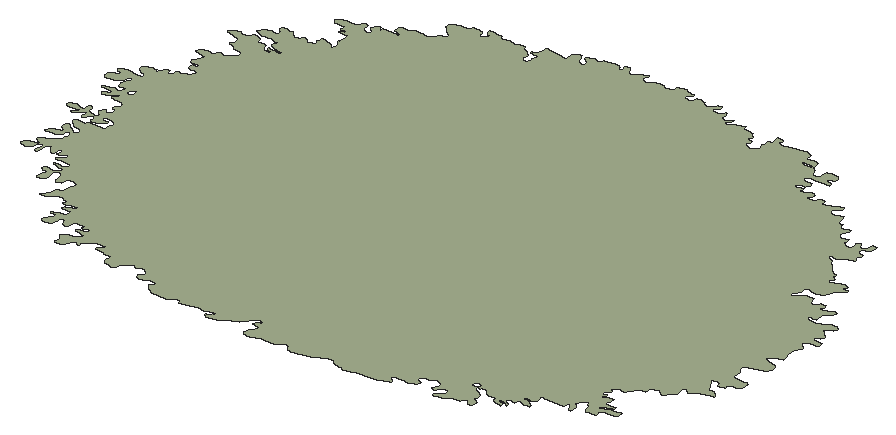
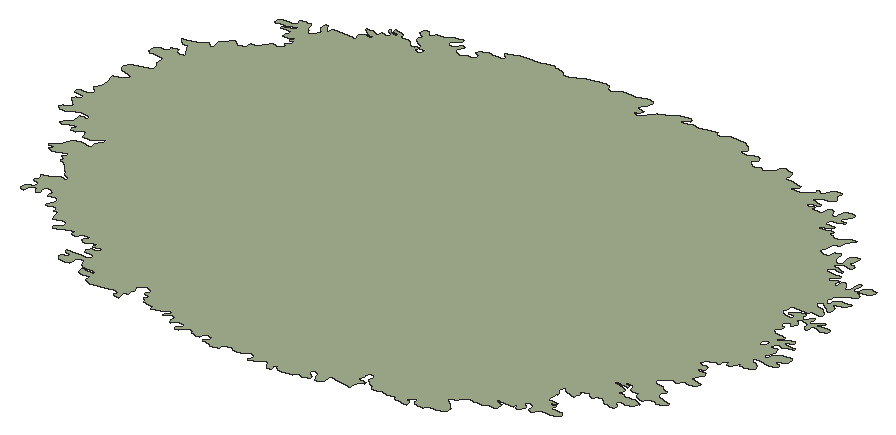
# SketchUp Ruby script. Lengths in inches.
U = 1.inch
M = Sketchup.active_model
def pt(a) = Geom::Point3d.new(a.map { |v| v * U })
def face(e, loops, mat)
  f = e.add_face(loops[0].map { |a| pt(a) })
  loops[1..].each { |l| e.add_face(l.map { |a| pt(a) }).erase! }
  f.material = f.back_material = mat if mat
  f
end
# faces: each face lists its corners as indices into pts; further lists are holes
def faces(e, pts, list, mat = nil) = list.each { |f| face(e, (f[0].is_a?(Array) ? f : [f]).map { |l| l.map { |i| pts[i] } }, mat) }
# xy, xz, yz: faces in a plane at the given z, y or x. An outline is a flat list of corners, or four numbers for a rectangle; further outlines are holes
def ring(l) = l.size == 4 ? [[l[0], l[1]], [l[2], l[1]], [l[2], l[3]], [l[0], l[3]]] : l.each_slice(2).to_a
def flat(e, list, mat, &to3) = list.each { |f| face(e, (f[0].is_a?(Array) ? f : [f]).map { |l| ring(l).map { |u, v| to3.(u, v) } }, mat) }
def xy(e, z, list, mat = nil) = flat(e, list, mat) { |x, y| [x, y, z] }
def xz(e, y, list, mat = nil) = flat(e, list, mat) { |x, z| [x, y, z] }
def yz(e, x, list, mat = nil) = flat(e, list, mat) { |y, z| [x, y, z] }
def lines(e, pts, list) = list.each { |a, b| e.add_line(pt(pts[a]), pt(pts[b])) }
# prism: a flat outline (further loops are holes) pulled along v
def prism(e, loops, v, mat = nil)
  f = face(e, loops, mat); d = Geom::Vector3d.new(v.map { |x| x * U })
  f.pushpull(f.normal.samedirection?(d) ? d.length : -d.length)
end
def box(e, o, s, mat = nil) = prism(e, [[o, [o[0] + s[0], o[1], o[2]], [o[0] + s[0], o[1] + s[1], o[2]], [o[0], o[1] + s[1], o[2]]]], [0, 0, s[2]], mat)
def at(x, y, z, deg = 0) = Geom::Transformation.translation(pt([x, y, z])) * Geom::Transformation.rotation(ORIGIN, Z_AXIS, deg.degrees)
def axes(o, x, y, z) = Geom::Transformation.new([*x, 0, *y, 0, *z, 0, *pt(o).to_a, 1])
def part(name) = M.definitions.add(name)
# library, detail: a bought-in or finely detailed component or shape, given as its bounding box
def library(name, o, s) = part(name).tap { |d| box(d.entities, o, s) }
def detail(e, o, s) = box(e.add_group.entities, o, s)
def put(e, d, t, mat = nil) = e.add_instance(d, t).tap { |i| i.material = mat if mat }
def group(e, t, mat = nil) = e.add_group.tap { |g| g.transformation = t; g.material = mat if mat }.entities
root = M.entities
M.materials.add("Boxwoodplan").color = [166, 177, 144]
xy(root,9.058,[[[245.938,66.701,245.827,66.705,245.732,66.73,245.676,66.786,245.675,66.889,245.701,66.953,245.764,67.016,245.813,67.08,245.872,67.177,245.685,67.207,245.595,67.216,245.615,67.304,245.701,67.362,245.732,67.372,245.727,67.417,245.638,67.449,245.522,67.408,245.425,67.278,245.283,67.123,245.122,67.036,245.016,67.013,244.956,66.988,244.94,66.945,244.795,66.853,244.602,66.822,244.513,66.831,244.432,66.878,244.432,66.899,244.478,66.93,244.568,67.008,244.637,67.055,244.547,67.069,244.435,67.052,244.315,67.007,244.121,67.025,244.024,67.018,243.898,66.974,243.697,66.928,243.608,66.92,243.57,67.014,243.5625,67.036,243.495,67.044,243.406,67.026,243.238,66.908,243.038,66.899,242.808,66.924,242.641,67.018,242.499,67.181,242.682,67.274,242.583,67.327,242.447,67.344,242.32,67.321,242.248,67.268,242.168,67.244,242.052,67.309,242.01,67.377,242.097,67.418,242.124,67.479,242.129,67.529,242.088,67.581,242.015,67.657,241.93,67.689,241.843,67.635,241.776,67.61,241.72,67.652,241.704,67.675,241.68,67.693,241.65,67.683,241.571,67.629,241.499,67.581,241.423,67.495,241.412,67.362,241.34,67.32,241.29,67.294,241.23,67.297,241.131,67.317,241.045,67.365,241.001,67.433,240.992,67.522,241.001,67.589,241.014,67.611,240.995,67.651,240.782,67.671,240.85,67.707,240.823,67.708,240.731,67.702,240.561,67.718,240.484,67.744,240.467,67.778,240.481,67.796,240.607,67.885,240.604,67.942,240.52,67.965,240.36,67.961,240.23,67.891,240.132,67.805,240.058,67.77,240.01,67.744,240.009,67.725,240.046,67.673,240.03,67.617,239.959,67.653,239.896,67.692,239.834,67.644,239.812,67.589,239.781,67.475,239.733,67.427,239.66,67.393,239.569,67.387,239.499,67.413,239.481,67.446,239.488,67.464,239.509,67.504,239.531,67.563,239.5,67.62,239.399,67.721,239.513,67.801,239.574,67.841,239.653,67.856,239.721,67.887,239.776,67.941,239.86,68.048,239.789,68.074,239.709,68.082,239.577,68.102,239.538,68.137,239.546,68.156,239.62,68.191,239.782,68.229,239.825,68.28,239.82,68.319,239.794,68.335,239.644,68.282,239.598,68.304,239.599,68.323,239.621,68.386,239.46,68.397,239.38,68.405,239.326,68.397,239.318,68.378,239.302,68.281,239.287,68.214,239.246,68.163,239.199,68.15,239.179,68.165,239.12,68.211,239.076,68.329,239.036,68.355,239.009,68.356,238.956,68.348,238.949,68.329,238.947,68.213,238.892,68.095,238.832,68.021,238.752,67.991,238.673,67.994,238.626,68.019,238.593,68.078,238.594,68.135,238.647,68.248,238.761,68.356,238.782,68.374,238.768,68.394,238.742,68.4,238.661,68.418,238.581,68.431,238.554,68.447,238.56,68.466,238.581,68.485,238.729,68.553,238.891,68.577,238.933,68.679,238.907,68.74,238.86,68.762,238.832,68.758,238.669,68.74,238.629,68.771,238.635,68.791,238.663,68.85,238.82,68.905,238.992,68.975,239.041,69.014,239.027,69.035,238.931,69.008,238.759,68.989,238.615,68.943,238.526,68.957,238.499,68.963,238.506,68.983,238.526,68.998,238.581,69.042,238.554,69.079,238.526,69.075,238.444,69.083,238.389,69.131,238.375,69.173,238.347,69.169,238.265,69.146,238.108,69.06,237.958,68.984,237.884,68.952,237.829,68.964,237.842,68.984,237.862,69.024,237.888,69.041,237.913,69.121,237.962,69.222,237.994,69.33,238.045,69.384,238.119,69.423,238.163,69.544,238.185,69.684,238.204,69.798,238.2,69.857,238.155,69.893,238.075,69.906,237.988,69.906,237.915,69.881,237.905,69.817,237.905,69.755,237.872,69.696,237.784,69.659,237.728,69.668,237.689,69.727,237.679,69.788,237.653,69.909,237.647,69.971,237.607,70.025,237.579,70.047,237.542,70.0625,237.483,70.051,237.448,70.031,237.447,70,237.439,69.938,237.441,69.801,237.466,69.739,237.458,69.675,237.408,69.61,237.359,69.582,237.321,69.57,237.284,69.575,237.242,69.583,237.224,69.61,237.22,69.738,237.241,69.795,237.286,69.848,237.302,69.878,237.293,69.906,237.236,69.911,237.155,69.918,237.117,69.933,237.094,69.962,237.091,70.024,237.107,70.055,237.141,70.071,237.314,70.043,237.392,70.068,237.442,70.098,237.502,70.145,237.516,70.208,237.493,70.234,237.449,70.235,237.371,70.242,237.279,70.253,237.178,70.289,237.16,70.318,237.165,70.332,237.185,70.335,237.244,70.347,237.42,70.333,237.509,70.358,237.522,70.415,237.496,70.478,237.424,70.518,237.345,70.524,237.231,70.518,237.132,70.492,237.048,70.51,237.044,70.54,237.065,70.568,237.111,70.625,237.178,70.682,237.231,70.762,237.222,70.796,237.178,70.8125,237.113,70.811,236.995,70.711,236.955,70.713,236.921,70.733,236.942,70.792,236.959,70.859,236.915,70.921,236.875,70.938,236.855,70.939,236.85,70.924,236.854,70.878,236.851,70.735,236.81,70.674,236.77,70.679,236.736,70.703,236.638,70.834,236.613,70.899,236.589,70.926,236.573,70.915,236.518,70.865,236.483,70.806,236.502,70.675,236.507,70.608,236.487,70.543,236.438,70.534,236.403,70.55,236.393,70.594,236.413,70.726,236.423,70.804,236.423,70.842,236.408,70.854,236.393,70.843,236.313,70.809,236.274,70.754,236.264,70.691,236.225,70.649,236.088,70.558,236.049,70.549,236.004,70.558,235.925,70.598,235.904,70.628,235.908,70.661,235.941,70.722,236.039,70.808,236.128,70.835,236.218,70.835,236.313,70.839,236.253,70.89,236.101,70.975,236.085,71.037,236.138,71.075,236.229,71.144,236.348,71.206,236.467,71.281,236.502,71.294,236.528,71.318,236.555,71.361,236.558,71.453,236.59,71.574,236.591,71.636,236.57,71.657,236.549,71.666,236.486,71.681,236.452,71.676,236.449,71.66,236.46,71.567,236.419,71.506,236.371,71.47,236.293,71.442,236.222,71.43,236.062,71.405,236.027,71.41,236.013,71.424,236.014,71.432,236.022,71.472,236.039,71.518,236.081,71.566,236.151,71.613,236.209,71.635,236.268,71.637,236.306,71.639,236.326,71.647,236.349,71.668,236.345,71.692,236.29,71.723,236.222,71.779,236.19,71.836,236.186,71.903,236.199,71.953,236.252,71.998,236.278,72.003,236.289,71.996,236.308,71.983,236.351,71.922,236.4,71.876,236.529,71.798,236.602,71.764,236.638,71.748,236.658,71.756,236.682,71.777,236.688,71.794,236.7,71.835,236.684,71.892,236.642,71.938,236.609,71.961,236.576,71.973,236.516,71.973,236.442,71.976,236.398,72.018,236.312,72.09,236.253,72.141,236.214,72.188,236.215,72.217,236.239,72.243,236.296,72.27,236.331,72.275,236.372,72.271,236.432,72.251,236.493,72.249,236.529,72.256,236.564,72.297,236.612,72.328,236.672,72.336,236.743,72.335,236.896,72.343,237.037,72.363,237.069,72.38,237.07,72.397,237.064,72.44,237.053,72.484,237.064,72.528,237.094,72.632,237.08,72.655,237.058,72.668,237.001,72.698,236.947,72.735,236.875,72.763,236.802,72.766,236.751,72.756,236.73,72.742,236.705,72.69,236.71,72.669,236.722,72.665,236.745,72.66,236.896,72.648,236.922,72.642,236.928,72.634,236.918,72.618,236.878,72.578,236.833,72.535,236.768,72.499,236.707,72.455,236.634,72.42,236.597,72.424,236.577,72.435,236.552,72.471,236.545,72.567,236.528,72.592,236.546,72.606,236.553,72.649,236.547,72.659,236.535,72.66,236.521,72.658,236.495,72.655,236.462,72.648,236.445,72.636,236.363,72.541,236.332,72.486,236.3,72.463,236.278,72.466,236.252,72.487,236.243,72.504,236.237,72.544,236.265,72.629,236.271,72.674,236.262,72.701,236.241,72.708,236.203,72.699,236.183,72.686,236.137,72.636,236.016,72.529,235.979,72.504,235.954,72.499,235.916,72.506,235.904,72.523,235.996,72.629,236.058,72.674,236.072,72.7,236.072,72.717,236.063,72.724,236.051,72.72,236.037,72.714,236.005,72.703,235.922,72.679,235.754,72.661,235.681,72.668,235.634,72.693,235.612,72.72,235.611,72.737,235.628,72.789,235.675,72.835,235.736,72.852,235.806,72.856,235.881,72.838,236.008,72.795,236.094,72.768,236.106,72.772,236.106,72.781,236.105,72.791,236.096,72.811,236.072,72.858,236.07,72.914,236.078,72.979,236.089,73.009,236.107,73.021,236.155,72.984,236.195,72.935,236.222,72.889,236.231,72.827,236.243,72.775,236.258,72.747,236.282,72.746,236.416,72.729,236.489,72.715,236.524,72.712,236.542,72.726,236.558,72.774,236.502,72.816,236.444,72.88,236.426,72.907,236.426,72.924,236.46,73.032,236.49,73.055,236.518,73.06,236.532,73.049,236.541,73.031,236.57,72.986,236.582,72.961,236.594,72.963,236.615,72.975,236.695,73.053,236.711,73.099,236.713,73.151,236.699,73.183,236.678,73.195,236.614,73.218,236.575,73.237,236.566,73.258,236.582,73.308,236.638,73.345,236.673,73.367,236.686,73.387,236.693,73.441,236.692,73.488,236.596,73.563,236.453,73.585,236.39,73.602,236.356,73.584,236.327,73.586,236.258,73.603,236.239,73.63,236.249,73.654,236.375,73.756,236.368,73.789,236.346,73.804,236.302,73.796,236.273,73.787,236.147,73.726,236.107,73.679,236.057,73.635,235.988,73.62,235.96,73.621,235.913,73.673,235.941,73.698,235.959,73.737,235.991,73.76,236.084,73.791,236.129,73.821,236.119,73.852,236.106,73.855,236.096,73.848,236.07,73.841,236.03,73.844,235.895,73.856,235.749,73.884,235.725,73.899,235.73,73.918,235.755,73.947,235.968,74.007,236.032,74.006,236.092,73.99,236.153,73.962,236.179,73.964,236.186,73.974,236.235,74.052,236.258,74.067,236.265,74.086,236.264,74.129,236.264,74.154,236.254,74.164,236.24,74.162,236.183,74.163,236.125,74.156,236.078,74.139,236.054,74.147,236.033,74.168,236.009,74.201,235.989,74.289,235.999,74.378,236.029,74.42,236.035,74.452,236.048,74.494,236.086,74.515,236.081,74.562,236.059,74.598,235.97,74.575,235.953,74.541,235.954,74.521,235.957,74.458,235.876,74.411,235.735,74.317,235.58,74.271,235.496,74.297,235.454,74.35,235.444,74.476,235.573,74.561,235.655,74.575,235.699,74.599,235.723,74.633,235.721,74.653,235.636,74.684,235.5625,74.71,235.5,74.766,235.536,74.82,235.612,74.849,235.708,74.883,235.773,74.882,235.951,74.839,236.043,74.817,236.128,74.821,236.179,74.84,236.185,74.861,236.17,74.927,236.109,74.979,236.064,74.986,235.952,75.057,235.905,75.099,235.89,75.135,235.884,75.189,235.884,75.216,235.897,75.231,235.939,75.266,235.99,75.281,236.104,75.312,236.134,75.322,236.175,75.321,236.225,75.317,236.237,75.305,236.252,75.275,236.267,75.261,236.276,75.261,236.305,75.264,236.321,75.276,236.341,75.326,236.369,75.359,236.386,75.382,236.388,75.407,236.405,75.432,236.424,75.444,236.472,75.456,236.511,75.448,236.533,75.404,236.537,75.353,236.553,75.326,236.575,75.326,236.616,75.367,236.641,75.41,236.656,75.514,236.671,75.539,236.704,75.546,236.735,75.546,236.755,75.534,236.776,75.512,236.808,75.511,236.86,75.533,236.905,75.579,236.918,75.603,236.908,75.617,236.968,75.615,236.996,75.618,237.012,75.637,237.017,75.686,237.051,75.726,237.086,75.772,237.032,75.815,236.964,75.844,236.927,75.842,236.895,75.832,236.852,75.821,236.811,75.827,236.789,75.843,236.767,75.866,236.744,75.969,236.757,75.994,236.763,76.011,236.773,76.014,236.877,76.035,236.923,76.043,236.942,76.054,236.932,76.058,236.846,76.086,236.78,76.098,236.752,76.091,236.716,76.091,236.68,76.092,236.645,76.104,236.606,76.154,236.588,76.183,236.588,76.213,236.604,76.235,236.632,76.25,236.664,76.269,236.672,76.296,236.701,76.354,236.729,76.408,236.735,76.461,236.727,76.488,236.687,76.499,236.609,76.525,236.436,76.572,236.401,76.59,236.384,76.614,236.419,76.668,236.464,76.703,236.509,76.73,236.564,76.75,236.617,76.759,236.669,76.756,236.724,76.732,236.78,76.734,236.806,76.738,236.819,76.759,236.837,76.8,236.874,76.836,236.894,76.854,236.921,76.856,236.99,76.839,237.052,76.828,237.078,76.825,237.102,76.84,237.188,76.907,237.276,76.972,237.329,77.069,237.326,77.114,237.284,77.15,237.167,77.188,237.042,77.218,236.955,77.291,236.898,77.326,236.829,77.347,236.801,77.359,236.788,77.38,236.81,77.426,236.858,77.468,236.856,77.553,236.806,77.631,236.676,77.6875,236.436,77.767,236.387,77.784,236.367,77.818,236.438,77.882,236.559,77.933,236.665,77.938,236.722,77.925,236.766,77.899,236.814,77.889,236.867,77.897,236.928,77.909,236.958,77.94,236.972,78.019,236.99,78.054,237.043,78.053,237.1,78.043,237.148,78.023,237.215,77.964,237.24,77.929,237.254,77.889,237.255,77.821,237.261,77.816,237.269,77.82,237.296,77.834,237.348,77.84,237.436,77.842,237.516,77.806,237.551,77.742,237.575,77.664,237.645,77.619,237.686,77.606,237.703,77.606,237.73,77.615,237.826,77.621,237.842,77.626,237.822,77.643,237.759,77.666,237.708,77.671,237.669,77.689,237.65,77.724,237.647,77.736,237.651,77.755,237.666,77.763,237.7,77.763,237.742,77.756,237.849,77.728,237.963,77.723,238.015,77.731,238.034,77.733,238.06,77.745,238.016,77.775,237.974,77.785,237.888,77.799,237.83,77.813,237.79,77.816,237.767,77.82,237.742,77.834,237.691,77.86,237.643,77.887,237.621,77.919,237.632,77.975,237.66,78.014,237.701,78.043,237.661,78.074,237.606,78.089,237.564,78.092,237.508,78.1,237.477,78.126,237.46,78.163,237.445,78.172,237.417,78.171,237.301,78.143,237.249,78.129,237.199,78.13,237.152,78.133,237.102,78.15,237.054,78.167,237.014,78.174,236.971,78.198,236.928,78.221,236.954,78.234,236.955,78.241,236.967,78.281,236.982,78.317,237.008,78.354,237.039,78.386,237.083,78.411,237.136,78.433,237.182,78.445,237.288,78.439,237.365,78.433,237.398,78.429,237.408,78.429,237.408,78.442,237.4,78.483,237.379,78.528,237.343,78.567,237.301,78.598,237.268,78.644,237.27,78.668,237.28,78.688,237.328,78.718,237.38,78.741,237.406,78.741,237.432,78.735,237.487,78.719,237.554,78.714,237.602,78.699,237.625,78.686,237.644,78.667,237.687,78.626,237.726,78.591,237.771,78.56,237.828,78.547,237.881,78.552,237.927,78.581,237.958,78.617,238.007,78.655,238.033,78.655,238.056,78.64,238.096,78.598,238.143,78.565,238.271,78.59,238.346,78.609,238.387,78.637,238.393,78.657,238.371,78.673,238.32,78.695,238.311,78.718,238.319,78.741,238.334,78.785,238.341,78.845,238.345,78.87,238.368,78.886,238.396,78.888,238.426,78.879,238.468,78.86,238.602,78.82,238.662,78.798,238.702,78.765,238.728,78.725,238.743,78.702,238.75,78.694,238.76,78.698,238.767,78.703,238.8,78.748,238.806,78.783,238.796,78.886,238.775,78.934,238.75,78.968,238.715,79.008,238.705,79.037,238.717,79.049,238.728,79.046,238.749,79.048,238.748,79.056,238.754,79.079,238.746,79.121,238.732,79.277,238.734,79.354,238.618,79.373,238.521,79.376,238.459,79.384,238.441,79.391,238.427,79.401,238.44,79.411,238.553,79.453,238.587,79.482,238.587,79.495,238.564,79.519,238.528,79.523,238.475,79.512,238.427,79.49,238.409,79.49,238.394,79.517,238.421,79.6,238.423,79.64,238.423,79.654,238.399,79.675,238.31,79.657,238.197,79.66,238.087,79.676,238.026,79.757,238.024,79.784,238.062,79.821,238.159,79.875,238.207,79.901,238.262,79.907,238.386,79.904,238.478,79.908,238.537,79.917,238.577,79.955,238.617,79.99,238.625,80.033,238.652,80.072,238.707,80.085,238.745,80.08,238.788,80.046,238.799,79.96,238.806,79.871,238.829,79.829,238.885,79.803,238.976,79.783,239.031,79.806,239.049,79.847,239.026,79.89,238.98,79.927,238.923,80.014,238.959,80.093,239.034,80.175,239.053,80.178,239.076,80.148,239.095,80.1,239.169,80.018,239.197,79.992,239.188,80.047,239.17,80.142,239.227,80.159,239.288,80.153,239.415,80.15,239.528,80.147,239.649,80.129,239.668,80.129,239.655,80.158,239.605,80.2,239.474,80.252,239.436,80.261,239.414,80.306,239.416,80.397,239.45,80.442,239.499,80.468,239.615,80.472,239.712,80.481,239.807,80.549,239.934,80.553,240.05,80.542,240.145,80.524,240.266,80.517,240.309,80.563,240.323,80.61,240.366,80.704,240.455,80.758,240.575,80.816,240.586,80.832,240.57,80.865,240.529,80.903,240.422,80.985,240.353,81.058,240.239,81.142,240.269,81.149,240.268,81.162,240.264,81.183,240.252,81.251,240.256,81.281,240.291,81.315,240.373,81.356,240.456,81.393,240.495,81.399,240.551,81.397,240.637,81.388,240.661,81.38,240.685,81.382,240.716,81.415,240.768,81.49,240.804,81.504,240.861,81.507,240.963,81.502,241.059,81.47,241.092,81.449,241.121,81.407,241.122,81.336,241.124,81.308,241.129,81.286,241.153,81.276,241.206,81.286,241.251,81.316,241.312,81.37,241.337,81.393,241.359,81.405,241.371,81.422,241.287,81.468,241.249,81.484,241.205,81.528,241.18,81.607,241.181,81.638,241.24,81.655,241.431,81.626,241.528,81.611,241.564,81.597,241.563,81.551,241.573,81.523,241.634,81.519,241.738,81.534,241.839,81.546,241.881,81.543,241.928,81.529,241.956,81.506,241.98,81.505,242.005,81.514,242.149,81.543,242.19,81.552,242.243,81.559,242.279,81.555,242.323,81.529,242.354,81.457,242.38,81.434,242.425,81.416,242.465,81.405,242.505,81.379,242.557,81.325,242.61,81.268,242.597,81.191,242.591,81.117,242.605,81.087,242.636,81.056,242.662,81.033,242.709,81.025,242.746,81.022,242.79,81.052,242.804,81.084,242.805,81.125,242.793,81.199,242.829,81.359,242.818,81.388,242.8,81.401,242.777,81.404,242.738,81.405,242.686,81.399,242.649,81.398,242.603,81.406,242.577,81.429,242.585,81.451,242.612,81.468,242.652,81.482,242.697,81.508,242.722,81.584,242.725,81.749,242.726,81.781,242.748,81.8,242.775,81.804,242.873,81.794,243.072,81.772,243.164,81.762,243.252,81.74,243.339,81.725,243.39,81.718,243.385,81.926,243.454,81.998,243.538,82.058,243.593,82.048,243.62,82.013,243.669,81.942,243.692,81.868,243.7,81.832,243.698,81.8125,243.725,81.778,243.83,81.745,243.881,81.744,243.92,81.776,243.923,81.851,243.821,81.931,243.743,81.99,243.755,82.024,243.799,82.061,243.892,82.112,243.942,82.121,244.023,82.109,244.128,82.109,244.15,82.187,244.36,82.215,244.461,82.233,244.568,82.218,244.647,82.15,244.681,82.115,244.707,82.112,244.747,82.139,244.745,82.215,244.737,82.257,244.749,82.291,244.8,82.3,244.855,82.286,244.926,82.193,244.947,82.119,244.98,82.084,245.028,82.07,245.079,82.074,245.126,82.102,245.214,82.185,245.295,82.239,245.397,82.286,245.445,82.271,245.458,82.235,245.407,82.164,245.381,82.129,245.389,82.087,245.477,82.029,245.577,82.014,245.628,82.023,245.677,82.07,245.756,82.138,245.87,82.153,245.985,82.125,246.017,82.095,246.093,82.064,246.194,82.082,246.275,82.136,246.275,82.249,246.333,82.292,246.446,82.316,246.551,82.311,246.632,82.252,246.778,82.232,246.831,82.222,246.837,82.185,246.764,82.118,246.731,82.045,246.743,82.008,246.814,81.968,246.917,81.972,246.969,82.005,246.989,82.044,247.01,82.116,247.058,82.139,247.082,82.15,247.134,82.15,247.237,82.112,247.28,82.041,247.365,81.988,247.496,82.018,247.53,82.049,247.537,82.092,247.576,82.175,247.683,82.193,247.713,82.163,247.719,82.122,247.667,82.038,247.618,82.02,247.591,81.985,247.652,81.92,247.782,81.908,247.873,81.944,247.941,82.015,247.965,82.022,247.974,82.004,247.993,81.964,248.017,81.929,248.005,81.872,247.986,81.829,248.004,81.794,248.093,81.751,248.201,81.756,248.256,81.774,248.306,81.829,248.323,81.845,248.326,81.826,248.312,81.784,248.24,81.704,248.206,81.673,248.217,81.638,248.264,81.619,248.321,81.619,248.418,81.66,248.5,81.717,248.719,81.796,248.741,81.725,248.764,81.694,248.816,81.69,248.931,81.682,249.055,81.656,249.07,81.584,249.093,81.554,249.14,81.536,249.163,81.501,249.148,81.464,249.122,81.366,249.238,81.345,249.284,81.326,249.295,81.291,249.221,81.222,249.206,81.184,249.223,81.15,249.298,81.098,249.402,81.072,249.503,81.067,249.615,81.135,249.657,81.21,249.599,81.282,249.566,81.351,249.586,81.456,249.595,81.493,249.565,81.527,249.562,81.563,249.603,81.59,249.704,81.594,249.693,81.693,249.652,81.845,249.701,81.859,249.766,81.846,249.819,81.828,249.851,81.771,249.801,81.703,249.804,81.666,249.851,81.648,249.958,81.648,250.088,81.682,250.596,81.749,250.641,81.74,250.6875,81.716,250.734,81.693,250.768,81.669,250.799,81.599,250.781,81.507,250.986,81.52,251.051,81.514,251.135,81.483,251.172,81.376,251.158,81.328,251.141,81.296,251.1,81.288,250.931,81.32,250.866,81.326,250.824,81.326,250.803,81.321,250.8,81.305,250.829,81.257,250.869,81.237,250.917,81.238,251.089,81.253,251.158,81.255,251.243,81.22,251.28,81.18,251.31,81.117,251.378,81.008,251.458,80.969,251.542,80.965,251.573,81.006,251.567,81.09,251.549,81.142,251.556,81.208,251.597,81.258,251.698,81.29,251.808,81.304,251.896,81.273,251.944,81.231,251.978,81.168,251.979,81.122,251.918,81.067,251.851,81.053,251.81,81.042,251.778,81.009,251.782,80.979,251.832,80.96,251.93,80.934,252.001,80.91,252.021,80.878,252.009,80.846,251.955,80.819,251.867,80.811,251.706,80.805,251.618,80.793,251.53,80.827,251.465,80.841,251.384,80.822,251.327,80.779,251.326,80.715,251.384,80.675,251.471,80.652,251.556,80.637,251.603,80.637,251.637,80.618,251.659,80.575,251.642,80.51,251.607,80.462,251.579,80.437,251.534,80.426,251.391,80.406,251.371,80.4,251.362,80.355,251.367,80.322,251.411,80.304,251.479,80.302,251.52,80.302,251.57,80.318,251.633,80.349,251.647,80.284,251.617,80.237,251.611,80.207,251.65,80.188,251.711,80.194,251.792,80.241,251.848,80.283,251.876,80.307,251.914,80.292,251.978,80.276,252.047,80.223,252.043,80.175,252,80.109,251.967,80.044,251.986,80.02,252.033,80.017,252.108,80.027,252.19,80.067,252.229,80.125,252.301,80.168,252.361,80.181,252.398,80.173,252.416,80.149,252.42,80.12,252.403,80.093,252.375,80.069,252.377,80.054,252.397,80.052,252.569,80.071,252.65,80.082,252.717,80.124,252.759,80.16,252.838,80.186,252.935,80.191,252.958,80.167,252.962,80.138,252.801,79.921,252.816,79.875,252.873,79.823,252.956,79.808,253.046,79.827,253.114,79.854,253.198,79.876,253.263,79.785,253.3,79.571,253.301,79.557,253.338,79.546,253.421,79.567,253.432,79.49,253.456,79.442,253.532,79.433,253.67,79.467,253.738,79.465,253.752,79.411,253.684,79.19,253.674,79.139,253.697,79.086,253.763,79.057,253.831,79.067,253.967,79.095,253.987,78.99,253.982,78.887,254.104,78.819,254.236,78.788,254.267,78.889,254.256,78.993,254.234,79.045,254.262,79.096,254.33,79.107,254.369,79.053,254.391,79,254.439,78.966,254.517,78.989,254.57,79.039,254.595,79.155,254.598,79.207,254.659,79.231,254.717,79.202,254.747,79.149,254.721,79.026,254.606,78.947,254.553,78.91,254.533,78.853,254.513,78.803,254.535,78.757,254.667,78.733,254.724,78.705,254.728,78.654,254.656,78.569,254.69,78.467,254.72,78.415,254.708,78.366,254.574,78.34,254.472,78.3,254.369,78.23,254.317,78.195,254.252,78.197,254.188,78.231,254.155,78.238,254.129,78.214,254.174,78.12,254.293,78.055,254.339,78.016,254.336,77.967,254.421,77.891,254.588,77.704,254.719,77.621,254.783,77.607,254.82,77.564,254.805,77.469,254.92,77.406,254.857,77.32,254.837,77.268,254.836,77.245,254.867,77.232,255.004,77.25,255.139,77.327,255.268,77.339,255.393,77.305,255.397,77.258,255.33,77.232,255.305,77.215,255.319,77.191,255.397,77.171,255.468,77.168,255.5,77.167,255.514,77.143,255.425,77.054,255.259,76.894,255.235,76.803,255.231,76.758,255.204,76.714,255.11,76.639,254.982,76.61,254.857,76.615,254.749,76.654,254.679,76.647,254.652,76.576,254.68,76.466,254.65,76.359,254.532,76.291,254.56,76.192,254.698,76.213,254.87,76.404,255.098,76.386,255.174,76.177,255.219,76.166,255.3,76.19,255.388,76.294,255.526,76.307,255.563,76.207,255.513,76.146,255.499,76.111,255.575,76.072,255.714,76.102,255.834,76.169,255.881,76.185,255.97,76.164,255.948,76.049,255.838,75.955,255.773,75.861,255.78,75.684,255.766,75.65,255.674,75.627,255.541,75.659,255.566,75.553,255.698,75.513,255.844,75.507,255.992,75.536,256.229,75.658,256.366,75.67,256.458,75.579,256.425,75.476,256.285,75.421,256.237,75.397,256.209,75.337,256.312,75.247,256.463,75.087,256.431,74.986,256.314,74.931,256.278,74.907,256.317,74.846,256.46,74.84,256.591,74.818,256.602,74.717,256.53,74.661,256.396,74.649,256.271,74.612,256.228,74.514,256.397,74.333,256.289,74.139,256.293,73.96,256.347,73.747,256.391,73.649,256.258,73.622,256.135,73.579,256.042,73.503,256.014,73.44,256.126,73.373,256.377,73.316,256.454,73.234,256.475,73.131,256.433,73.039,256.319,72.965,255.858,72.805,255.859,72.713,255.903,72.619,255.957,72.526,255.959,72.434,255.95,72.344,255.976,72.29,256.097,72.248,256.222,72.243,256.349,72.253,256.39,72.252,256.448,72.204,256.459,72.025,256.432,71.966,256.323,71.919,256.197,71.901,256.156,71.903,256.109,71.853,256.152,71.763,256.138,71.734,256.054,71.715,256.013,71.717,255.943,71.742,255.91,71.831,255.841,71.863,255.717,71.868,255.675,71.862,255.66,71.804,255.735,71.728,255.822,71.564,255.851,71.541,255.877,71.489,255.894,71.459,255.975,71.449,256.056,71.431,256.141,71.363,256.204,71.282,256.201,71.253,256.116,71.228,255.868,71.187,255.672,71.059,255.599,71.041,255.505,71.116,255.465,71.124,255.401,71.091,255.404,71.006,255.46,70.842,255.418,70.835,255.384,70.791,255.335,70.751,255.282,70.638,255.243,70.59,255.208,70.571,255.173,70.585,255.05,70.671,254.988,70.686,254.945,70.688,254.9,70.669,254.837,70.635,254.807,70.5625,254.816,70.509,254.798,70.445,254.637,70.424,254.584,70.382,254.552,70.331,254.506,70.289,254.494,70.226,254.463,70.181,254.429,70.154,254.391,70.144,254.322,70.135,254.224,70.147,254.164,70.122,254.103,70.074,254.073,70.028,254.147,69.991,254.174,69.948,254.138,69.892,254.084,69.856,254.063,69.796,254.062,69.781,254.06,69.766,254.08,69.758,254.151,69.751,254.177,69.754,254.197,69.753,254.201,69.738,254.164,69.668,254.144,69.621,254.141,69.591,254.182,69.59,254.322,69.666,254.39,69.682,254.471,69.679,254.455,69.575,254.438,69.462,254.438,69.414,254.461,69.392,254.501,69.39,254.564,69.417,254.645,69.417,254.704,69.404,254.744,69.399,254.751,69.369,254.711,69.331,254.632,69.302,254.565,69.293,254.482,69.268,254.443,69.23,254.427,69.173,254.43,69.159,254.47,69.157,254.553,69.183,254.71,69.245,254.864,69.275,254.99,69.277,255.043,69.257,255.018,69.183,254.997,69.141,254.935,69.09,254.783,69.064,254.643,69.062,254.583,69.054,254.552,68.999,254.577,68.88,254.562,68.835,254.481,68.814,254.345,68.827,254.287,68.832,254.243,68.886,254.235,68.997,254.234,69.039,254.222,69.068,254.214,69.082,254.194,69.083,254.135,69.096,254.131,69.153,254.132,69.167,254.129,69.181,254.109,69.186,254.029,69.189,253.972,69.163,253.928,69.108,253.89,69.07,253.866,69.012,253.876,68.962,253.932,68.926,254.007,68.826,254.003,68.727,253.995,68.687,253.987,68.66,253.956,68.637,253.937,68.638,253.915,68.669,253.886,68.728,253.821,68.83,253.78,68.869,253.767,68.884,253.756,68.87,253.749,68.843,253.746,68.798,253.727,68.745,253.721,68.731,253.691,68.715,253.607,68.708,253.467,68.71,253.18,68.711,253.123,68.734,253.036,68.744,253.016,68.735,253.01,68.705,253.061,68.645,253.086,68.547,253.079,68.508,253.048,68.468,253.023,68.46,252.963,68.452,252.86,68.452,252.763,68.456,252.714,68.424,252.77,68.4,252.87,68.385,252.978,68.352,253.053,68.298,253.134,68.225,253.116,68.201,253.056,68.185,252.955,68.193,252.917,68.201,252.867,68.221,252.818,68.256,252.768,68.28,252.733,68.201,252.724,68.13,252.683,68.117,252.627,68.13,252.583,68.16,252.57,68.172,252.551,68.179,252.54,68.162,252.506,68.085,252.507,68.056,252.541,68.019,252.633,67.988,252.671,67.954,252.685,67.912,252.683,67.898,252.663,67.895,252.621,67.932,252.541,67.981,252.447,67.998,252.39,68,252.379,67.987,252.4,67.961,252.514,67.918,252.55,67.906,252.574,67.864,252.568,67.822,252.525,67.82,252.413,67.832,252.308,67.867,252.273,67.896,252.264,67.942,252.262,68.012,252.212,68.032,252.152,68.013,252.052,68.021,251.954,68.039,251.927,68.061,251.902,68.097,251.906,68.14,251.912,68.154,251.874,68.163,251.78,68.188,251.741,68.189,251.722,68.19,251.687,68.177,251.675,68.149,251.656,68.143,251.629,68.169,251.625,68.183,251.656,68.207,251.671,68.217,251.664,68.243,251.576,68.3,251.539,68.324,251.52,68.328,251.44,68.288,251.42,68.281,251.408,68.253,251.431,68.162,251.527,68.158,251.565,68.153,251.596,68.113,251.589,68.085,251.583,68.071,251.59,68.042,251.702,68.006,251.789,67.967,251.851,67.909,251.867,67.884,251.866,67.87,251.832,67.854,251.812,67.845,251.843,67.823,251.897,67.796,251.909,67.772,251.859,67.739,251.847,67.712,251.872,67.677,251.957,67.633,252.034,67.566,252.034,67.422,252.012,67.396,251.96,67.385,251.906,67.401,251.869,67.445,251.828,67.51,251.811,67.521,251.773,67.516,251.72,67.498,251.699,67.468,251.7,67.425,251.699,67.412,251.665,67.4,251.489,67.39,251.48,67.397,251.433,67.379,251.389,67.348,251.305,67.263,251.252,67.233,251.179,67.223,251.041,67.215,250.987,67.23,250.984,67.269,251.093,67.333,251.194,67.405,251.191,67.508,251.184,67.552,251.185,67.565,251.153,67.587,251.094,67.606,251.019,67.605,250.936,67.521,250.916,67.482,250.858,67.438,250.844,67.429,250.807,67.437,250.771,67.451,250.758,67.478,250.799,67.57,250.858,67.666,250.86,67.706,250.792,67.76,250.68,67.795,250.629,67.818,250.591,67.809,250.567,67.786,250.533,67.743,250.5,67.727,250.458,67.729,250.402,67.738,250.364,67.739,250.326,67.717,250.246,67.622,250.259,67.581,250.333,67.541,250.388,67.509,250.416,67.488,250.425,67.461,250.401,67.423,250.34,67.379,250.239,67.327,250.183,67.307,250.11,67.309,250.055,67.331,249.982,67.341,249.936,67.316,249.9,67.314,249.868,67.332,249.8125,67.337,249.74,67.324,249.717,67.289,249.728,67.23,249.824,67.146,249.852,67.107,249.852,67.069,249.834,67.063,249.544,66.963,249.269,66.941,249.036,66.944,248.946,66.942,248.823,66.881,248.72,66.847,248.623,66.851,248.586,66.852,248.536,66.87,248.488,66.9,248.428,66.897,248.339,66.905,248.255,66.947,248.195,67.004,248.163,67.05,248.105,67.063,248.005,67.05,247.91,67.01,247.829,66.969,247.73,66.896,247.633,66.84,247.54,66.811,247.299,66.793,247.109,66.757,247.013,66.761,246.948,66.856,246.917,66.922,246.828,66.937,246.737,66.924,246.641,66.851,246.576,66.789,246.486,66.782,246.31,66.805,246.124,66.812,246.046,66.761],[236.446,73.986,236.489,73.991,236.508,73.993,236.534,74.002,236.546,74.045,236.547,74.084,236.554,74.169,236.546,74.202,236.534,74.215,236.535,74.229,236.491,74.206,236.435,74.184,236.416,74.177,236.4,74.161,236.378,74.129,236.369,74.091,236.371,74.047,236.39,74.009,236.408,73.993]]],"Boxwoodplan")
